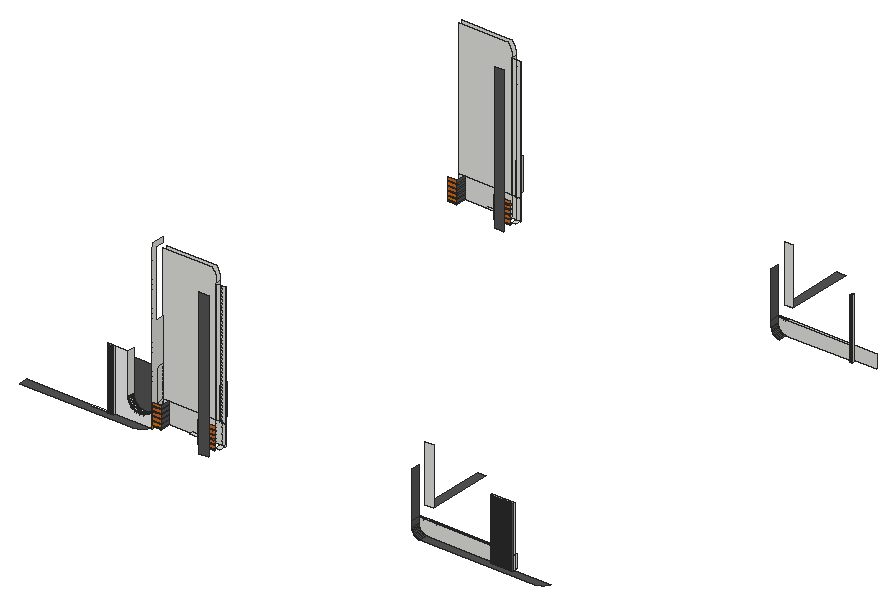
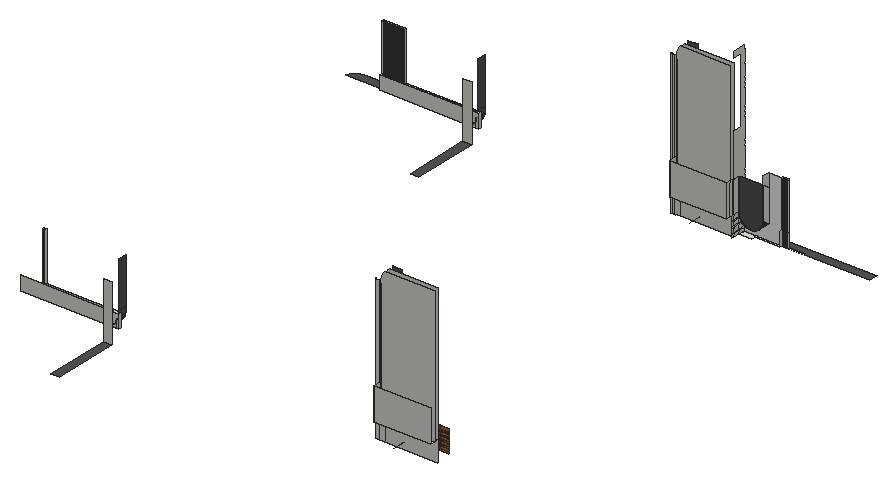
# SketchUp Ruby script. Lengths in inches.
U = 1.inch
M = Sketchup.active_model
def pt(a) = Geom::Point3d.new(a.map { |v| v * U })
def face(e, loops, mat)
  f = e.add_face(loops[0].map { |a| pt(a) })
  loops[1..].each { |l| e.add_face(l.map { |a| pt(a) }).erase! }
  f.material = f.back_material = mat if mat
  f
end
# faces: each face lists its corners as indices into pts; further lists are holes
def faces(e, pts, list, mat = nil) = list.each { |f| face(e, (f[0].is_a?(Array) ? f : [f]).map { |l| l.map { |i| pts[i] } }, mat) }
# xy, xz, yz: faces in a plane at the given z, y or x. An outline is a flat list of corners, or four numbers for a rectangle; further outlines are holes
def ring(l) = l.size == 4 ? [[l[0], l[1]], [l[2], l[1]], [l[2], l[3]], [l[0], l[3]]] : l.each_slice(2).to_a
def flat(e, list, mat, &to3) = list.each { |f| face(e, (f[0].is_a?(Array) ? f : [f]).map { |l| ring(l).map { |u, v| to3.(u, v) } }, mat) }
def xy(e, z, list, mat = nil) = flat(e, list, mat) { |x, y| [x, y, z] }
def xz(e, y, list, mat = nil) = flat(e, list, mat) { |x, z| [x, y, z] }
def yz(e, x, list, mat = nil) = flat(e, list, mat) { |y, z| [x, y, z] }
def lines(e, pts, list) = list.each { |a, b| e.add_line(pt(pts[a]), pt(pts[b])) }
# prism: a flat outline (further loops are holes) pulled along v
def prism(e, loops, v, mat = nil)
  f = face(e, loops, mat); d = Geom::Vector3d.new(v.map { |x| x * U })
  f.pushpull(f.normal.samedirection?(d) ? d.length : -d.length)
end
def box(e, o, s, mat = nil) = prism(e, [[o, [o[0] + s[0], o[1], o[2]], [o[0] + s[0], o[1] + s[1], o[2]], [o[0], o[1] + s[1], o[2]]]], [0, 0, s[2]], mat)
def at(x, y, z, deg = 0) = Geom::Transformation.translation(pt([x, y, z])) * Geom::Transformation.rotation(ORIGIN, Z_AXIS, deg.degrees)
def axes(o, x, y, z) = Geom::Transformation.new([*x, 0, *y, 0, *z, 0, *pt(o).to_a, 1])
def part(name) = M.definitions.add(name)
# library, detail: a bought-in or finely detailed component or shape, given as its bounding box
def library(name, o, s) = part(name).tap { |d| box(d.entities, o, s) }
def detail(e, o, s) = box(e.add_group.entities, o, s)
def put(e, d, t, mat = nil) = e.add_instance(d, t).tap { |i| i.material = mat if mat }
def group(e, t, mat = nil) = e.add_group.tap { |g| g.transformation = t; g.material = mat if mat }.entities
root = M.entities
M.materials.add("[0039_DarkOrange]").color = [219, 120, 0]
M.materials.add("[0041_Chocolate]").color = [210, 105, 30]
M.materials.add("[0129_WhiteSmoke]").color = [245, 245, 245]
M.materials.add("[Color M06]").color = [84, 84, 84]
xy(root,141.26,[[1486.5,281.47,1527.09,285.84],[1527.09,281.47,1545.07,281.47,1545.83,283,1546.87,286.06,1547.5,289.23,1547.71,292.45,1527.09,292.45],[1545.07,281.47,1545.83,283,1546.87,286.06,1547.5,289.23,1547.71,292.45,1547.71,281.47],[1976.54,281.47,1993.98,285.84],[1993.98,281.47,2137,285.84],
  [1642.35,292.45,1649.14,302.46],[2008.98,972.36,2026.42,976.74],[1570.66,983.34,1577.46,993.35]])
xy(root,141.26,[[1343.48,267.75,1523.01,267.75,1526.23,267.96,1529.4,268.59,1532.46,269.63,1535.36,271.06,1538.05,272.85,1540.48,274.98,1542.61,277.41,1544.4,280.1,1545.07,281.47,1486.5,281.47,1486.5,278.34,1483.38,278.34,1483.38,281.47,1482.13,281.47,1482.13,278.34,1479,278.34,1479,281.47,1477.94,281.47,1477.94,278.34,1474.82,278.34,1474.82,281.47,1473.75,281.47,1473.75,278.34,1470.63,278.34,1470.63,281.47,1469.57,281.47,1469.57,278.34,1466.44,278.34,1466.44,281.47,1465.38,281.47,1465.38,278.34,1462.25,278.34,1462.25,281.47,1461.13,281.47,1461.13,278.34,1458,278.34,1458,281.47,1456.88,281.47,1456.88,278.34,1453.75,278.34,1453.75,281.47,1452.63,281.47,1452.63,278.34,1449.5,278.34,1449.5,281.47,1343.48,281.47],[1993.98,267.75,2173.51,267.75,2176.73,267.96,2179.9,268.59,2182.96,269.63,2185.86,271.06,2188.55,272.85,2190.98,274.98,2193.11,277.41,2194.9,280.1,2195.57,281.47,2137,281.47,2137,278.34,2133.88,278.34,2133.88,281.47,2132.63,281.47,2132.63,278.34,2129.5,278.34,2129.5,281.47,2128.44,281.47,2128.44,278.34,2125.32,278.34,2125.32,281.47,2124.25,281.47,2124.25,278.34,2121.13,278.34,2121.13,281.47,2120.07,281.47,2120.07,278.34,2116.94,278.34,2116.94,281.47,2115.88,281.47,2115.88,278.34,2112.75,278.34,2112.75,281.47,2111.63,281.47,2111.63,278.34,2108.5,278.34,2108.5,281.47,2107.38,281.47,2107.38,278.34,2104.25,278.34,2104.25,281.47,2103.13,281.47,2103.13,278.34,2100,278.34,2100,281.47,1993.98,281.47]],"[Color M06]")
xy(root,145.27,[[1597.48,295.65,1622.67,300.34],[1525.8,986.55,1550.98,991.24]])
xy(root,145.27,[[1547.71,280.47,1563.1,281.47],[1476.02,971.36,1491.41,972.36]],"[0039_DarkOrange]")
xy(root,145.27,[[1622.67,280.47,1649.14,281.47],[1550.98,971.36,1577.46,972.36]],"[0041_Chocolate]")
xy(root,147.375,[[1547.71,280.47,1563.1,281.47],[1476.02,971.36,1491.41,972.36]],"[0039_DarkOrange]")
xy(root,147.375,[[1622.67,280.47,1649.14,281.47],[1550.98,971.36,1577.46,972.36]],"[0041_Chocolate]")
xy(root,148.66,[[1949.9,333.33,1963.61,439.98],[1982.33,1024.22,1996.05,1130.875]],"[Color M06]")
xy(root,152.33,[[1547.71,280.47,1563.1,281.47],[1476.02,971.36,1491.41,972.36]],"[0039_DarkOrange]")
xy(root,152.33,[[1622.67,280.47,1649.14,281.47],[1550.98,971.36,1577.46,972.36]],"[0041_Chocolate]")
xy(root,154.4375,[[1547.71,280.47,1563.1,281.47],[1622.67,280.47,1649.14,281.47],[1476.02,971.36,1491.41,972.36],[1550.98,971.36,1577.46,972.36]],"[0041_Chocolate]")
xy(root,159.39,[[1547.71,280.47,1563.1,281.47],[1622.67,280.47,1649.14,281.47],[1476.02,971.36,1491.41,972.36],[1550.98,971.36,1577.46,972.36]],"[0041_Chocolate]")
xy(root,161.5,[[1547.71,280.47,1563.1,281.47],[1622.67,280.47,1649.14,281.47],[1476.02,971.36,1491.41,972.36],[1550.98,971.36,1577.46,972.36]],"[0041_Chocolate]")
xy(root,163.7,[[1976.54,281.47,1993.98,285.84],[1993.98,281.47,2137,285.84],[2008.98,972.36,2026.42,976.74]])
xy(root,166.45,[[1547.71,280.47,1563.1,281.47],[1622.67,280.47,1649.14,281.47],[1476.02,971.36,1491.41,972.36],[1550.98,971.36,1577.46,972.36]],"[0041_Chocolate]")
xy(root,168.5625,[[1547.71,280.47,1563.1,281.47],[1622.67,280.47,1649.14,281.47],[1476.02,971.36,1491.41,972.36],[1550.98,971.36,1577.46,972.36]],"[0041_Chocolate]")
xy(root,173.52,[[1547.71,280.47,1563.1,281.47],[1622.67,280.47,1649.14,281.47],[1476.02,971.36,1491.41,972.36],[1550.98,971.36,1577.46,972.36]],"[0041_Chocolate]")
xy(root,174.51,[[1547.71,302.46,1634.68,310.27],[1634.68,302.46,1634.68,310.27,1547.71,310.27,1547.71,317.3125,1640.52,317.3125,1640.52,302.46],[1476.02,993.35,1562.99,1001.16],[1562.99,993.35,1562.99,1001.16,1476.02,1001.16,1476.02,1008.21,1568.84,1008.21,1568.84,993.35]])
xy(root,175.625,[[1547.71,280.47,1563.1,281.47],[1622.67,280.47,1649.14,281.47],[1476.02,971.36,1491.41,972.36],[1550.98,971.36,1577.46,972.36]],"[0041_Chocolate]")
xz(root,267.75,[[1634.68,141.3,1650.02,376.875]],"[Color M06]")
xz(root,278.34,[[1479,141.26,1482.13,240.16],[1483.38,141.26,1486.5,240.16],[2100,141.26,2103.13,240.16],[2104.25,141.26,2107.38,240.16],[2108.5,141.26,2111.63,240.16],
  [2112.75,141.26,2115.88,240.16],[2116.94,141.26,2120.07,240.16],[2121.13,141.26,2124.25,240.16],[2125.32,141.26,2128.44,240.16],[2129.5,141.26,2132.63,240.16],
  [2133.88,141.26,2137,240.16]],"[Color M06]")
xz(root,280.47,[[1547.71,147.375,1563.1,152.33]],"[0039_DarkOrange]")
xz(root,280.47,[[1622.67,147.375,1649.14,152.33],[1547.71,154.4375,1563.1,159.39],[1622.67,154.4375,1649.14,159.39],[1547.71,161.5,1563.1,166.45],[1622.67,161.5,1649.14,166.45],
  [1547.71,168.5625,1563.1,173.52],[1622.67,168.5625,1649.14,173.52],[1547.71,175.625,1563.1,180.58],[1622.67,175.625,1649.14,180.58]],"[0041_Chocolate]")
xz(root,281.47,[[1474.82,141.26,1477.94,163.7],[1477.94,141.26,1479,163.7],[1479,141.26,1482.13,163.7],[1482.13,141.26,1483.38,163.7],[1483.38,141.26,1486.5,163.7],
  [1976.54,141.26,1980.54,163.7],[1980.54,141.26,1993.98,141.26,1992.2,141.46,1990.46,141.89,1988.79,142.53,1987.21,143.38,1985.75,144.42,1984.43,145.64,1983.28,147.01,1982.32,148.52,1981.55,150.14,1980.99,151.84,1980.65,153.6,1980.54,155.39],[1993.98,141.26,2100,141.26,2100,163.7,1980.54,163.7,1980.54,155.39,1980.65,153.6,1980.99,151.84,1981.55,150.14,1982.32,148.52,1983.28,147.01,1984.43,145.64,1985.75,144.42,1987.21,143.38,1988.79,142.53,1990.46,141.89,1992.2,141.46],[2100,141.26,2103.13,163.7],[2103.13,141.26,2104.25,163.7],
  [2104.25,141.26,2107.38,163.7],[2107.38,141.26,2108.5,163.7],[2108.5,141.26,2111.63,163.7],[2111.63,141.26,2112.75,163.7],[2112.75,141.26,2115.88,163.7],
  [2115.88,141.26,2116.94,163.7],[2116.94,141.26,2120.07,163.7],[2120.07,141.26,2121.13,163.7],[2121.13,141.26,2124.25,163.7],[2124.25,141.26,2125.32,163.7],
  [2125.32,141.26,2128.44,163.7],[2128.44,141.26,2129.5,163.7],[2129.5,141.26,2132.63,163.7],[2132.63,141.26,2133.88,163.7],[2133.88,141.26,2137,163.7],
  [1474.82,163.7,1477.94,240.16],[1479,163.7,1482.13,240.16],[1483.38,163.7,1486.5,240.16],[2100,163.7,2103.13,240.16],[2104.25,163.7,2107.38,240.16],
  [2108.5,163.7,2111.63,240.16],[2112.75,163.7,2115.88,240.16],[2116.94,163.7,2120.07,240.16],[2121.13,163.7,2124.25,240.16],[2125.32,163.7,2128.44,240.16],
  [2129.5,163.7,2132.63,240.16],[2133.88,163.7,2137,240.16]])
xz(root,281.47,[[1547.71,145.27,1563.1,147.375]],"[0039_DarkOrange]")
xz(root,281.47,[[1622.67,145.27,1649.14,147.375],[1547.71,152.33,1563.1,154.4375],[1622.67,152.33,1649.14,154.4375],[1547.71,159.39,1563.1,161.5],[1622.67,159.39,1649.14,161.5],
  [1547.71,166.45,1563.1,168.5625],[1622.67,166.45,1649.14,168.5625],[1547.71,173.52,1563.1,175.625],[1622.67,173.52,1649.14,175.625]],"[0041_Chocolate]")
xz(root,281.47,[[1486.5,141.26,1547.71,141.26,1547.71,174.51,1547.68,173.46,1547.6,172.42,1547.46,171.38,1547.27,170.36,1547.03,169.34,1546.73,168.33,1546.38,167.35,1545.98,166.38,1545.53,165.4375,1545.03,164.52,1544.49,163.625,1543.89,162.76,1543.26,161.93,1542.58,161.14,1541.86,160.38,1541.1,159.66,1540.3,158.98,1539.47,158.34,1538.61,157.75,1537.72,157.2,1536.8,156.7,1535.86,156.25,1534.89,155.85,1533.9,155.5,1532.9,155.21,1531.88,154.96,1530.85,154.77,1529.82,154.64,1528.77,154.55,1527.73,154.53,1526.68,154.55,1525.64,154.64,1524.6,154.77,1523.57,154.96,1522.55,155.21,1521.55,155.5,1520.57,155.85,1519.6,156.25,1518.65,156.7,1517.73,157.2,1516.84,157.75,1515.98,158.34,1515.15,158.98,1514.35,159.66,1513.6,160.38,1512.875,161.14,1512.2,161.93,1511.56,162.76,1510.97,163.625,1510.42,164.52,1509.92,165.4375,1509.47,166.38,1509.07,167.35,1508.72,168.33,1508.42,169.34,1508.18,170.36,1507.99,171.38,1507.85,172.42,1507.77,173.46,1507.74,174.51,1507.74,240.16,1486.5,240.16]],"[0129_WhiteSmoke]")
xz(root,285.84,[[1976.54,141.26,1976.54,163.7,1993.98,163.7,1993.98,141.26,1992.2,141.46,1990.46,141.89,1988.79,142.53,1987.21,143.38,1985.75,144.42,1984.43,145.64,1983.28,147.01,1982.32,148.52,1981.55,150.14,1980.99,151.84,1980.65,153.6,1980.54,155.39,1980.54,141.26],[1980.54,141.26,1980.54,155.39,1980.65,153.6,1980.99,151.84,1981.55,150.14,1982.32,148.52,1983.28,147.01,1984.43,145.64,1985.75,144.42,1987.21,143.38,1988.79,142.53,1990.46,141.89,1992.2,141.46,1993.98,141.26],[1993.98,141.26,2137,163.7]])
xz(root,292.45,[[1498.09,174.51,1507.74,226.8]])
xz(root,292.45,[[1527.73,154.53,1528.77,154.55,1529.82,154.64,1530.85,154.77,1531.88,154.96,1532.9,155.21,1533.9,155.5,1534.89,155.85,1535.86,156.25,1536.8,156.7,1537.72,157.2,1538.61,157.75,1539.47,158.34,1540.3,158.98,1541.1,159.66,1541.86,160.38,1542.58,161.14,1543.26,161.93,1543.89,162.76,1544.49,163.625,1545.03,164.52,1545.53,165.4375,1545.98,166.38,1546.38,167.35,1546.73,168.33,1547.03,169.34,1547.27,170.36,1547.46,171.38,1547.6,172.42,1547.68,173.46,1547.71,174.51,1547.71,226.8,1507.74,226.8,1507.74,174.51,1507.77,173.46,1507.85,172.42,1507.99,171.38,1508.18,170.36,1508.42,169.34,1508.72,168.33,1509.07,167.35,1509.47,166.38,1509.92,165.4375,1510.42,164.52,1510.97,163.625,1511.56,162.76,1512.2,161.93,1512.875,161.14,1513.6,160.38,1514.35,159.66,1515.15,158.98,1515.98,158.34,1516.84,157.75,1517.73,157.2,1518.65,156.7,1519.6,156.25,1520.57,155.85,1521.55,155.5,1522.55,155.21,1523.57,154.96,1524.6,154.77,1525.64,154.64,1526.68,154.55]],"[Color M06]")
xz(root,302.46,[[1547.71,141.26,1634.68,174.51],[1634.68,141.26,1643.23,174.51],[1643.23,141.26,1649.14,174.51],[1649.14,141.26,1650.02,174.51],[1547.71,174.51,1634.68,174.51,1634.68,376.875,1634.67,377.55,1634.64,378.22,1634.6,378.9,1634.54,379.57,1634.46,380.24,1634.36,380.9,1634.25,381.57,1634.12,382.23,1633.97,382.89,1633.8,383.54,1633.78,383.64,1633.62,384.19,1633.42,384.84,1633.2,385.47,1633.1,385.76,1632.97,386.11,1632.72,386.73,1632.45,387.35,1632.17,387.96,1631.87,388.57,1631.56,389.17,1631.23,389.76,1630.88,390.33,1630.52,390.9,1630.15,391.47,1629.76,392.02,1629.36,392.56,1628.9375,393.09,1628.9,393.14,1628.51,393.6,1628.0625,394.11,1627.6,394.61,1627.13,395.09,1626.96,395.26,1547.71,395.26],
  [1634.68,174.51,1640.52,374.14],[1640.52,174.51,1643.23,374.14],[1643.23,174.51,1649.14,374.14],[1649.14,174.51,1650.02,374.14]])
xz(root,310.27,[[1547.71,174.51,1547.71,395.26,1626.96,395.26,1627.13,395.09,1627.6,394.61,1628.0625,394.11,1628.51,393.6,1628.9,393.14,1628.9375,393.09,1629.36,392.56,1629.76,392.02,1630.15,391.47,1630.52,390.9,1630.88,390.33,1631.23,389.76,1631.56,389.17,1631.87,388.57,1632.17,387.96,1632.45,387.35,1632.72,386.73,1632.97,386.11,1633.1,385.76,1633.2,385.47,1633.42,384.84,1633.62,384.19,1633.78,383.64,1633.8,383.54,1633.97,382.89,1634.12,382.23,1634.25,381.57,1634.36,380.9,1634.46,380.24,1634.54,379.57,1634.6,378.9,1634.64,378.22,1634.67,377.55,1634.68,376.875,1634.68,174.51]])
xz(root,317.3125,[[1547.71,174.51,1640.52,226.8]])
xz(root,333.33,[[1949.9,148.66,1963.61,240.16]])
xz(root,958.64,[[1562.99,141.3,1578.33,376.875]],"[Color M06]")
xz(root,969.24,[[2132.44,141.26,2135.57,240.16]],"[Color M06]")
xz(root,971.36,[[1476.02,147.375,1491.41,152.33]],"[0039_DarkOrange]")
xz(root,971.36,[[1550.98,147.375,1577.46,152.33],[1476.02,154.4375,1491.41,159.39],[1550.98,154.4375,1577.46,159.39],[1476.02,161.5,1491.41,166.45],[1550.98,161.5,1577.46,166.45],
  [1476.02,168.5625,1491.41,173.52],[1550.98,168.5625,1577.46,173.52],[1476.02,175.625,1491.41,180.58],[1550.98,175.625,1577.46,180.58]],"[0041_Chocolate]")
xz(root,972.36,[[2008.98,141.26,2012.97,163.7],[2012.97,141.26,2026.42,141.26,2024.64,141.46,2022.9,141.89,2021.22,142.53,2019.64,143.38,2018.1875,144.42,2016.87,145.64,2015.72,147.01,2014.75,148.52,2013.98,150.14,2013.43,151.84,2013.09,153.6,2012.97,155.39],[2026.42,141.26,2132.44,141.26,2132.44,163.7,2012.97,163.7,2012.97,155.39,2013.09,153.6,2013.43,151.84,2013.98,150.14,2014.75,148.52,2015.72,147.01,2016.87,145.64,2018.1875,144.42,2019.64,143.38,2021.22,142.53,2022.9,141.89,2024.64,141.46],[2132.44,141.26,2135.57,163.7],[2135.57,141.26,2136.69,163.7],
  [2132.44,163.7,2135.57,240.16]])
xz(root,972.36,[[1476.02,145.27,1491.41,147.375]],"[0039_DarkOrange]")
xz(root,972.36,[[1550.98,145.27,1577.46,147.375],[1476.02,152.33,1491.41,154.4375],[1550.98,152.33,1577.46,154.4375],[1476.02,159.39,1491.41,161.5],[1550.98,159.39,1577.46,161.5],
  [1476.02,166.45,1491.41,168.5625],[1550.98,166.45,1577.46,168.5625],[1476.02,173.52,1491.41,175.625],[1550.98,173.52,1577.46,175.625]],"[0041_Chocolate]")
xz(root,976.74,[[2008.98,141.26,2008.98,163.7,2026.42,163.7,2026.42,141.26,2024.64,141.46,2022.9,141.89,2021.22,142.53,2019.64,143.38,2018.1875,144.42,2016.87,145.64,2015.72,147.01,2014.75,148.52,2013.98,150.14,2013.43,151.84,2013.09,153.6,2012.97,155.39,2012.97,141.26],[2012.97,141.26,2012.97,155.39,2013.09,153.6,2013.43,151.84,2013.98,150.14,2014.75,148.52,2015.72,147.01,2016.87,145.64,2018.1875,144.42,2019.64,143.38,2021.22,142.53,2022.9,141.89,2024.64,141.46,2026.42,141.26],[2026.42,141.26,2169.44,163.7]])
xz(root,993.35,[[1476.02,141.26,1562.99,174.51],[1562.99,141.26,1571.54,174.51],[1571.54,141.26,1577.46,174.51],[1577.46,141.26,1578.33,174.51],[1476.02,174.51,1562.99,174.51,1562.99,376.875,1562.98,377.55,1562.96,378.22,1562.91,378.9,1562.85,379.57,1562.77,380.24,1562.67,380.9,1562.56,381.57,1562.43,382.23,1562.28,382.89,1562.11,383.54,1562.09,383.64,1561.93,384.19,1561.73,384.84,1561.51,385.47,1561.41,385.76,1561.28,386.11,1561.03,386.73,1560.76,387.35,1560.48,387.96,1560.18,388.57,1559.87,389.17,1559.54,389.76,1559.2,390.33,1558.84,390.9,1558.46,391.47,1558.07,392.02,1557.67,392.56,1557.25,393.09,1557.21,393.14,1556.82,393.6,1556.375,394.11,1555.92,394.61,1555.45,395.09,1555.27,395.26,1476.02,395.26],
  [1562.99,174.51,1568.84,374.14],[1568.84,174.51,1571.54,374.14],[1571.54,174.51,1577.46,374.14],[1577.46,174.51,1578.33,374.14]])
xz(root,1001.16,[[1476.02,174.51,1476.02,395.26,1555.27,395.26,1555.45,395.09,1555.92,394.61,1556.375,394.11,1556.82,393.6,1557.21,393.14,1557.25,393.09,1557.67,392.56,1558.07,392.02,1558.46,391.47,1558.84,390.9,1559.2,390.33,1559.54,389.76,1559.87,389.17,1560.18,388.57,1560.48,387.96,1560.76,387.35,1561.03,386.73,1561.28,386.11,1561.41,385.76,1561.51,385.47,1561.73,384.84,1561.93,384.19,1562.09,383.64,1562.11,383.54,1562.28,382.89,1562.43,382.23,1562.56,381.57,1562.67,380.9,1562.77,380.24,1562.85,379.57,1562.91,378.9,1562.96,378.22,1562.98,377.55,1562.99,376.875,1562.99,174.51]])
xz(root,1008.21,[[1476.02,174.51,1568.84,226.8]])
xz(root,1024.22,[[1982.33,148.66,1996.05,240.16]])
yz(root,1477.94,[[278.34,141.26,281.47,240.16]])
yz(root,1479,[[278.34,141.26,281.47,240.16]])
yz(root,1482.13,[[278.34,141.26,281.47,240.16]])
yz(root,1483.38,[[278.34,141.26,281.47,240.16]])
yz(root,1486.5,[[278.34,141.26,281.47,240.16],[281.47,141.26,285.84,163.7]])
yz(root,1491.41,[[972.36,145.27,986.55,147.375],[971.36,147.375,986.55,152.33],[972.36,152.33,986.55,154.4375],[971.36,154.4375,986.55,159.39],[972.36,159.39,986.55,161.5],
  [971.36,161.5,986.55,166.45],[972.36,166.45,986.55,168.5625],[971.36,168.5625,986.55,173.52],[972.36,173.52,986.55,175.625],[971.36,175.625,986.55,180.58]],"[Color M06]")
yz(root,1507.74,[[281.47,174.51,292.45,240.16]])
yz(root,1547.71,[[281.47,141.26,292.45,146.14],[292.45,141.26,302.46,146.14],[302.46,141.26,305.58,146.14],[281.47,146.14,292.45,148.26],[292.45,146.14,302.46,148.26],
  [302.46,146.14,305.58,148.26],[281.47,148.26,292.45,155.64],[292.45,148.26,302.46,155.64],[302.46,148.26,305.58,155.64],[281.47,155.64,292.45,157.76],
  [292.45,155.64,302.46,157.76],[302.46,155.64,305.58,157.76],[281.47,157.76,292.45,165.14],[292.45,157.76,302.46,165.14],[302.46,157.76,305.58,165.14],
  [281.47,165.14,292.45,167.26],[292.45,165.14,302.46,167.26],[302.46,165.14,305.58,167.26],[281.47,167.26,292.45,174.51],[292.45,167.26,302.46,174.51],
  [302.46,167.26,305.58,174.51],[281.47,174.51,281.47,175.625,280.47,175.625,280.47,180.58,281.47,180.58,281.47,182.6875,280.47,182.6875,280.47,187.64,281.47,187.64,281.47,189.75,280.47,189.75,280.47,194.7,281.47,194.7,281.47,196.8125,280.47,196.8125,280.47,201.77,281.47,201.77,281.47,203.875,280.47,203.875,280.47,208.83,281.47,208.83,281.47,210.9375,280.47,210.9375,280.47,215.89,281.47,215.89,281.47,218,280.47,218,280.47,222.95,281.47,222.95,281.47,225.0625,280.47,225.0625,280.47,230.02,281.47,230.02,281.47,232.125,280.47,232.125,280.47,237.08,281.47,237.08,281.47,239.1875,280.47,239.1875,280.47,244.14,281.47,244.14,281.47,246.25,280.47,246.25,280.47,251.2,281.47,251.2,281.47,253.3125,280.47,253.3125,280.47,258.27,281.47,258.27,281.47,260.375,280.47,260.375,280.47,265.33,281.47,265.33,281.47,267.4375,280.47,267.4375,280.47,272.39,281.47,272.39,281.47,274.5,280.47,274.5,280.47,279.45,281.47,279.45,281.47,281.5625,280.47,281.5625,280.47,286.52,281.47,286.52,281.47,288.625,280.47,288.625,280.47,293.58,281.47,293.58,281.47,295.6875,280.47,295.6875,280.47,300.64,281.47,300.64,281.47,302.75,280.47,302.75,280.47,307.7,281.47,307.7,281.47,309.8125,280.47,309.8125,280.47,314.77,281.47,314.77,281.47,316.875,280.47,316.875,280.47,321.83,281.47,321.83,281.47,323.9375,280.47,323.9375,280.47,328.89,281.47,328.89,281.47,331,280.47,331,280.47,335.95,281.47,335.95,281.47,338.0625,280.47,338.0625,280.47,343.02,281.47,343.02,281.47,345.125,280.47,345.125,280.47,350.08,281.47,350.08,281.47,352.1875,280.47,352.1875,280.47,357.14,281.47,357.14,281.47,359.25,280.47,359.25,280.47,364.2,281.47,364.2,281.47,366.3125,280.47,366.3125,280.47,371.27,281.47,371.27,281.47,373.1875,280.47,373.1875,280.47,378.14,281.47,378.14,281.47,380.0625,280.47,380.0625,280.47,385.02,281.47,385.02,281.47,386.9375,280.47,386.9375,280.47,391.89,281.47,391.89,281.47,393.8125,280.47,393.8125,280.47,398.77,281.47,398.77,281.47,400.6875,280.47,400.6875,280.47,405.64,281.47,405.64,281.47,411.82,302.46,411.82,302.46,402.64,287.95,402.64,287.95,295.72,302.0625,295.72,302.0625,226.8,292.45,226.8,292.45,174.51],[292.45,174.51,302.46,226.8],[302.46,174.51,305.58,226.8],[305.58,174.51,310.27,226.8],
  [310.27,174.51,317.3125,226.8]])
yz(root,1547.71,[[280.47,141.26,281.47,145.27],[280.47,147.375,281.47,148.26],[280.47,148.26,281.47,152.33]],"[0039_DarkOrange]")
yz(root,1547.71,[[280.47,154.4375,281.47,155.64],[280.47,155.64,281.47,157.76],[280.47,157.76,281.47,159.39],[280.47,161.5,281.47,165.14],[280.47,165.14,281.47,166.45],
  [280.47,168.5625,281.47,173.52]],"[0041_Chocolate]")
yz(root,1550.98,[[972.36,145.27,986.55,147.375],[971.36,147.375,986.55,152.33],[972.36,152.33,986.55,154.4375],[971.36,154.4375,986.55,159.39],[972.36,159.39,986.55,161.5],
  [971.36,161.5,986.55,166.45],[972.36,166.45,986.55,168.5625],[971.36,168.5625,986.55,173.52],[972.36,173.52,986.55,175.625],[971.36,175.625,986.55,180.58]],"[Color M06]")
yz(root,1562.99,[[993.35,174.51,1001.16,374.14]])
yz(root,1563.1,[[281.47,145.27,295.65,147.375],[280.47,147.375,295.65,152.33],[281.47,152.33,295.65,154.4375],[280.47,154.4375,295.65,159.39],[281.47,159.39,295.65,161.5],
  [280.47,161.5,295.65,166.45],[281.47,166.45,295.65,168.5625],[280.47,168.5625,295.65,173.52],[281.47,173.52,295.65,175.625],[280.47,175.625,295.65,180.58]],"[Color M06]")
yz(root,1568.84,[[993.35,174.51,1008.21,226.8]])
yz(root,1622.67,[[281.47,145.27,295.65,147.375],[280.47,147.375,295.65,152.33],[281.47,152.33,295.65,154.4375],[280.47,154.4375,295.65,159.39],[281.47,159.39,295.65,161.5],
  [280.47,161.5,295.65,166.45],[281.47,166.45,295.65,168.5625],[280.47,168.5625,295.65,173.52],[281.47,173.52,295.65,175.625],[280.47,175.625,295.65,180.58]],"[Color M06]")
yz(root,1634.68,[[302.46,174.51,310.27,374.14]])
yz(root,1640.52,[[302.46,174.51,317.3125,226.8]])
yz(root,1976.54,[[281.47,141.26,285.84,163.7]])
yz(root,1980.54,[[267.75,155.39,281.47,164.97],[267.75,164.97,281.47,240.16]],"[Color M06]")
yz(root,2008.98,[[972.36,141.26,976.74,163.7]])
yz(root,2012.97,[[958.64,155.39,972.36,164.97],[958.64,164.97,972.36,240.16]],"[Color M06]")
yz(root,2100,[[278.34,141.26,281.47,240.16]])
yz(root,2103.13,[[278.34,141.26,281.47,240.16]])
yz(root,2104.25,[[278.34,141.26,281.47,240.16]])
yz(root,2107.38,[[278.34,141.26,281.47,240.16]])
yz(root,2108.5,[[278.34,141.26,281.47,240.16]])
yz(root,2111.63,[[278.34,141.26,281.47,240.16]])
yz(root,2112.75,[[278.34,141.26,281.47,240.16]])
yz(root,2115.88,[[278.34,141.26,281.47,240.16]])
yz(root,2116.94,[[278.34,141.26,281.47,240.16]])
yz(root,2120.07,[[278.34,141.26,281.47,240.16]])
yz(root,2121.13,[[278.34,141.26,281.47,240.16]])
yz(root,2124.25,[[278.34,141.26,281.47,240.16]])
yz(root,2125.32,[[278.34,141.26,281.47,240.16]])
yz(root,2128.44,[[278.34,141.26,281.47,240.16]])
yz(root,2129.5,[[278.34,141.26,281.47,240.16]])
yz(root,2132.44,[[969.24,141.26,972.36,240.16]])
yz(root,2132.63,[[278.34,141.26,281.47,240.16]])
yz(root,2133.88,[[278.34,141.26,281.47,240.16]])
yz(root,2135.57,[[969.24,141.26,972.36,240.16]])
yz(root,2136.69,[[969.24,141.26,972.36,240.16]])
p = [[1992.2,267.75,141.46],[1993.98,267.75,141.26],[1993.98,281.47,141.26],[1992.2,281.47,141.46],[1993.98,285.84,141.26],[1992.2,285.84,141.46],
  [2024.64,958.64,141.46],[2026.42,958.64,141.26],[2026.42,972.36,141.26],[2024.64,972.36,141.46],[2026.42,976.74,141.26],[2024.64,976.74,141.46],
  [1990.46,267.75,141.89],[1990.46,281.47,141.89],[1990.46,285.84,141.89],[2022.9,958.64,141.89],[2022.9,972.36,141.89],[2022.9,976.74,141.89],
  [1988.79,267.75,142.53],[1988.79,281.47,142.53],[1988.79,285.84,142.53],[2021.22,958.64,142.53],[2021.22,972.36,142.53],[2021.22,976.74,142.53],
  [1987.21,267.75,143.38],[1987.21,281.47,143.38],[1987.21,285.84,143.38],[2019.64,958.64,143.38],[2019.64,972.36,143.38],[2019.64,976.74,143.38],
  [1985.75,267.75,144.42],[1985.75,281.47,144.42],[1985.75,285.84,144.42],[2018.1875,958.64,144.42],[2018.1875,972.36,144.42],[2018.1875,976.74,144.42],
  [1984.43,267.75,145.64],[1984.43,281.47,145.64],[1984.43,285.84,145.64],[2016.87,958.64,145.64],[2016.87,972.36,145.64],[2016.87,976.74,145.64],
  [1983.28,267.75,147.01],[1983.28,281.47,147.01],[1983.28,285.84,147.01],[2015.72,958.64,147.01],[2015.72,972.36,147.01],[2015.72,976.74,147.01],
  [1982.32,267.75,148.52],[1982.32,281.47,148.52],[1982.32,285.84,148.52],[2014.75,958.64,148.52],[2014.75,972.36,148.52],[2014.75,976.74,148.52],
  [1981.55,267.75,150.14],[1981.55,281.47,150.14],[1981.55,285.84,150.14],[2013.98,958.64,150.14],[2013.98,972.36,150.14],[2013.98,976.74,150.14],
  [1980.99,267.75,151.84],[1980.99,281.47,151.84],[1980.99,285.84,151.84],[2013.43,958.64,151.84],[2013.43,972.36,151.84],[2013.43,976.74,151.84],
  [1980.65,267.75,153.6],[1980.65,281.47,153.6],[1980.65,285.84,153.6],[2013.09,958.64,153.6],[2013.09,972.36,153.6],[2013.09,976.74,153.6],
  [1980.54,267.75,155.39],[1980.54,281.47,155.39],[1980.54,285.84,155.39],[2012.97,958.64,155.39],[2012.97,972.36,155.39],[2012.97,976.74,155.39],
  [1527.73,292.45,154.53],[1526.68,292.45,154.55],[1526.68,281.47,154.55],[1527.73,281.47,154.53],[1528.77,292.45,154.55],[1528.77,281.47,154.55],
  [1525.64,292.45,154.64],[1524.6,292.45,154.77],[1524.6,281.47,154.77],[1525.64,281.47,154.64],[1529.82,292.45,154.64],[1529.82,281.47,154.64],
  [1530.85,292.45,154.77],[1530.85,281.47,154.77],[1523.57,292.45,154.96],[1523.57,281.47,154.96],[1531.88,292.45,154.96],[1531.88,281.47,154.96],
  [1522.55,292.45,155.21],[1522.55,281.47,155.21],[1532.9,292.45,155.21],[1532.9,281.47,155.21],[1521.55,292.45,155.5],[1521.55,281.47,155.5],
  [1533.9,292.45,155.5],[1533.9,281.47,155.5],[1520.57,292.45,155.85],[1520.57,281.47,155.85],[1534.89,292.45,155.85],[1534.89,281.47,155.85],
  [1519.6,292.45,156.25],[1519.6,281.47,156.25],[1535.86,292.45,156.25],[1535.86,281.47,156.25],[1518.65,292.45,156.7],[1518.65,281.47,156.7],
  [1536.8,292.45,156.7],[1536.8,281.47,156.7],[1517.73,292.45,157.2],[1517.73,281.47,157.2],[1537.72,292.45,157.2],[1537.72,281.47,157.2],
  [1516.84,292.45,157.75],[1516.84,281.47,157.75],[1538.61,292.45,157.75],[1538.61,281.47,157.75],[1515.98,292.45,158.34],[1515.98,281.47,158.34],
  [1539.47,292.45,158.34],[1539.47,281.47,158.34],[1515.15,292.45,158.98],[1515.15,281.47,158.98],[1540.3,292.45,158.98],[1540.3,281.47,158.98],
  [1514.35,292.45,159.66],[1514.35,281.47,159.66],[1541.1,292.45,159.66],[1541.1,281.47,159.66],[1513.6,292.45,160.38],[1513.6,281.47,160.38],
  [1541.86,292.45,160.38],[1541.86,281.47,160.38],[1512.875,292.45,161.14],[1512.875,281.47,161.14],[1542.58,292.45,161.14],[1542.58,281.47,161.14],
  [1512.2,292.45,161.93],[1512.2,281.47,161.93],[1543.26,292.45,161.93],[1543.26,281.47,161.93],[1511.56,292.45,162.76],[1511.56,281.47,162.76],
  [1543.89,292.45,162.76],[1543.89,281.47,162.76],[1510.97,292.45,163.625],[1510.97,281.47,163.625],[1544.49,292.45,163.625],[1544.49,281.47,163.625],
  [1510.42,292.45,164.52],[1510.42,281.47,164.52],[1545.03,292.45,164.52],[1545.03,281.47,164.52],[1509.92,292.45,165.4375],[1509.92,281.47,165.4375],
  [1545.53,292.45,165.4375],[1545.53,281.47,165.4375],[1509.47,292.45,166.38],[1509.47,281.47,166.38],[1545.98,292.45,166.38],[1545.98,281.47,166.38],
  [1509.07,292.45,167.35],[1509.07,281.47,167.35],[1546.38,292.45,167.35],[1546.38,281.47,167.35],[1508.72,292.45,168.33],[1508.72,281.47,168.33],
  [1546.73,292.45,168.33],[1546.73,281.47,168.33],[1508.42,292.45,169.34],[1508.42,281.47,169.34],[1547.03,292.45,169.34],[1547.03,281.47,169.34],
  [1508.18,292.45,170.36],[1508.18,281.47,170.36],[1547.27,292.45,170.36],[1547.27,281.47,170.36],[1507.99,292.45,171.38],[1507.99,281.47,171.38],
  [1547.46,292.45,171.38],[1547.46,281.47,171.38],[1507.85,292.45,172.42],[1507.85,281.47,172.42],[1547.6,292.45,172.42],[1547.6,281.47,172.42],
  [1507.77,292.45,173.46],[1507.77,281.47,173.46],[1547.68,292.45,173.46],[1547.68,281.47,173.46],[1507.74,292.45,174.51],[1507.74,281.47,174.51],
  [1547.71,292.45,174.51],[1547.71,281.47,174.51],[1588.26,321.34,165.14],[1588.26,343.15,165.14],[1516.57,1012.23,165.14],[1516.57,1034.04,165.14]]
faces(root,p,[[0,1,2,3],[6,7,8,9],[12,0,3,13],[15,6,9,16],[18,12,13,19],[21,15,16,22],[24,18,19,25],[27,21,22,28],
  [30,24,25,31],[33,27,28,34],[36,30,31,37],[39,33,34,40],[42,36,37,43],[45,39,40,46],[48,42,43,49],[51,45,46,52],
  [54,48,49,55],[57,51,52,58],[60,54,55,61],[63,57,58,64],[66,60,61,67],[69,63,64,70],[72,66,67,73],[75,69,70,76]],"[Color M06]")
faces(root,p,[[3,2,4,5],[9,8,10,11],[13,3,5,14],[16,9,11,17],[19,13,14,20],[22,16,17,23],[25,19,20,26],[28,22,23,29],
  [31,25,26,32],[34,28,29,35],[37,31,32,38],[40,34,35,41],[43,37,38,44],[46,40,41,47],[49,43,44,50],[52,46,47,53],
  [55,49,50,56],[58,52,53,59],[61,55,56,62],[64,58,59,65],[67,61,62,68],[70,64,65,71],[73,67,68,74],[76,70,71,77],
  [78,79,80,81],[82,78,81,83],[84,85,86,87],[79,84,87,80],[88,82,83,89],[90,88,89,91],[85,92,93,86],[94,90,91,95],
  [92,96,97,93],[98,94,95,99],[96,100,101,97],[102,98,99,103],[100,104,105,101],[106,102,103,107],[104,108,109,105],[110,106,107,111],
  [108,112,113,109],[114,110,111,115],[112,116,117,113],[118,114,115,119],[116,120,121,117],[122,118,119,123],[120,124,125,121],[126,122,123,127],
  [124,128,129,125],[130,126,127,131],[128,132,133,129],[134,130,131,135],[132,136,137,133],[138,134,135,139],[136,140,141,137],[142,138,139,143],
  [140,144,145,141],[146,142,143,147],[144,148,149,145],[150,146,147,151],[148,152,153,149],[154,150,151,155],[152,156,157,153],[158,154,155,159],
  [156,160,161,157],[162,158,159,163],[160,164,165,161],[166,162,163,167],[164,168,169,165],[170,166,167,171],[168,172,173,169],[174,170,171,175],
  [172,176,177,173],[178,174,175,179],[176,180,181,177],[182,178,179,183],[180,184,185,181],[186,182,183,187],[184,188,189,185],[190,186,187,191],
  [188,192,193,189],[194,190,191,195],[192,196,197,193],[198,194,195,199]])
lines(root,p,[[200,201],[202,203]])
